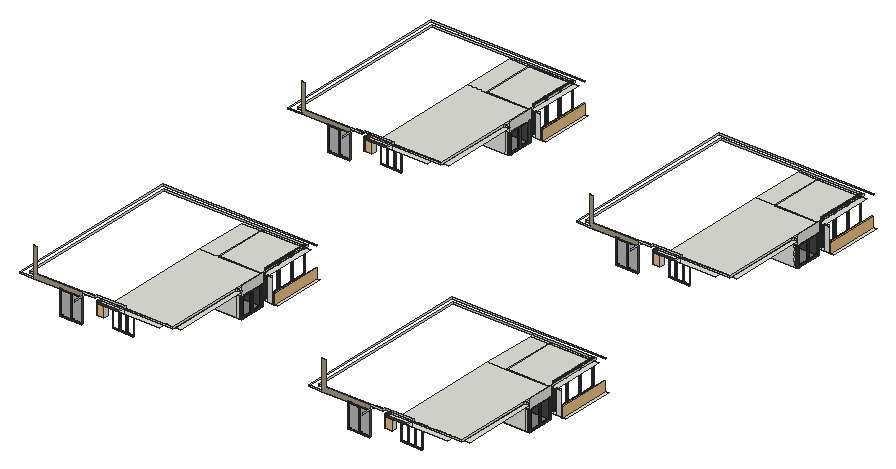
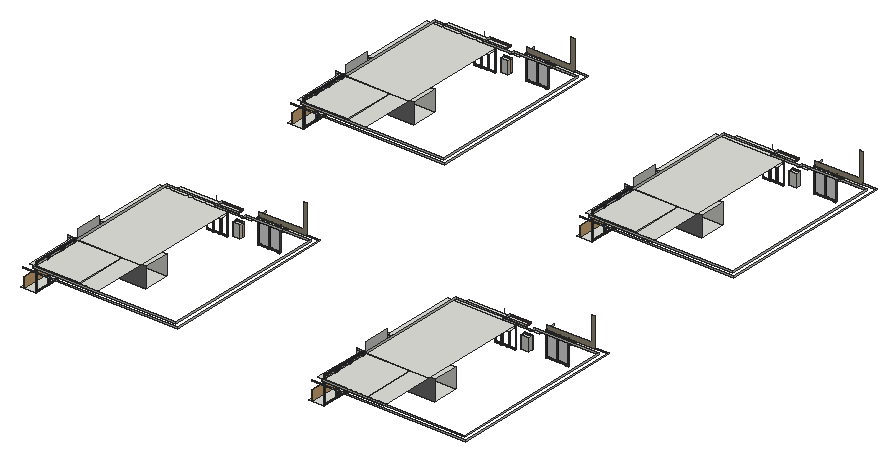
# SketchUp Ruby script. Lengths in inches.
U = 1.inch
M = Sketchup.active_model
def pt(a) = Geom::Point3d.new(a.map { |v| v * U })
def face(e, loops, mat)
  f = e.add_face(loops[0].map { |a| pt(a) })
  loops[1..].each { |l| e.add_face(l.map { |a| pt(a) }).erase! }
  f.material = f.back_material = mat if mat
  f
end
# faces: each face lists its corners as indices into pts; further lists are holes
def faces(e, pts, list, mat = nil) = list.each { |f| face(e, (f[0].is_a?(Array) ? f : [f]).map { |l| l.map { |i| pts[i] } }, mat) }
# xy, xz, yz: faces in a plane at the given z, y or x. An outline is a flat list of corners, or four numbers for a rectangle; further outlines are holes
def ring(l) = l.size == 4 ? [[l[0], l[1]], [l[2], l[1]], [l[2], l[3]], [l[0], l[3]]] : l.each_slice(2).to_a
def flat(e, list, mat, &to3) = list.each { |f| face(e, (f[0].is_a?(Array) ? f : [f]).map { |l| ring(l).map { |u, v| to3.(u, v) } }, mat) }
def xy(e, z, list, mat = nil) = flat(e, list, mat) { |x, y| [x, y, z] }
def xz(e, y, list, mat = nil) = flat(e, list, mat) { |x, z| [x, y, z] }
def yz(e, x, list, mat = nil) = flat(e, list, mat) { |y, z| [x, y, z] }
def lines(e, pts, list) = list.each { |a, b| e.add_line(pt(pts[a]), pt(pts[b])) }
# prism: a flat outline (further loops are holes) pulled along v
def prism(e, loops, v, mat = nil)
  f = face(e, loops, mat); d = Geom::Vector3d.new(v.map { |x| x * U })
  f.pushpull(f.normal.samedirection?(d) ? d.length : -d.length)
end
def box(e, o, s, mat = nil) = prism(e, [[o, [o[0] + s[0], o[1], o[2]], [o[0] + s[0], o[1] + s[1], o[2]], [o[0], o[1] + s[1], o[2]]]], [0, 0, s[2]], mat)
def at(x, y, z, deg = 0) = Geom::Transformation.translation(pt([x, y, z])) * Geom::Transformation.rotation(ORIGIN, Z_AXIS, deg.degrees)
def axes(o, x, y, z) = Geom::Transformation.new([*x, 0, *y, 0, *z, 0, *pt(o).to_a, 1])
def part(name) = M.definitions.add(name)
# library, detail: a bought-in or finely detailed component or shape, given as its bounding box
def library(name, o, s) = part(name).tap { |d| box(d.entities, o, s) }
def detail(e, o, s) = box(e.add_group.entities, o, s)
def put(e, d, t, mat = nil) = e.add_instance(d, t).tap { |i| i.material = mat if mat }
def group(e, t, mat = nil) = e.add_group.tap { |g| g.transformation = t; g.material = mat if mat }.entities
root = M.entities
M.materials.add("Glass_Tinted_Gray").color = [0, 0, 0]
M.materials["Glass_Tinted_Gray"].alpha = 0.125
M.materials.add("Wine2").color = [0, 0, 0]
M.materials["Wine2"].alpha = 0
M.materials.add("[0130_Gainsboro]").color = [39, 45, 50]
M.materials.add("[0135_DarkGray]").color = [81, 81, 81]
M.materials.add("[Color M05]").color = [114, 114, 114]
M.materials.add("[Color M06]").color = [86, 86, 86]
M.materials.add("[Concrete Tile]").color = [165, 155, 133]
M.materials.add("[Granite Brown]").color = [89, 59, 61]
M.materials.add("[Mirror 02]").color = [229, 229, 229]
M.materials.add("[Terrazzo Light Blue]").color = [196, 214, 227]
c1 = part("PENTEK_RP Fineline 50S_Sliding_DoorCase_E1")
box(c1.entities,[0,0,0],[1.51,3.66,99.27],"[0135_DarkGray]")
c2 = part("PENTEK_RP Fineline 50S_SlidingDooe_Case_E2")
box(c2.entities,[0,0,0],[96.25,3.66,1.51],"[0135_DarkGray]")
c3 = part("pentek_RP Fineline 50S_SlidingDoor_Case")
put(c3.entities,c1,at(97.76,0,0))
put(c3.entities,c2,at(1.51,0,0))
put(c3.entities,c1,at(0,0,0))
put(c3.entities,c2,at(1.51,0,97.76))
c4 = part("PENTEK_RP Fineline 50S_SlidingDoor_GlazingBead_2")
box(c4.entities,[0,0,0],[0.56,0.59,94.39],"[0135_DarkGray]")
c5 = part("PENTEK_RP Fineline 50S_SlidingDoor_Glass")
box(c5.entities,[0,0,0],[46.58,0.16,94.39],"Glass_Tinted_Gray")
c6 = part("PENTEK_RP Fineline 50S_SlidingDoor_GlazingBead")
box(c6.entities,[0,0,0],[45.47,0.59,0.56],"[0135_DarkGray]")
c7 = part("PENTEK_RP Fineline 50S_SlidingDoor_Leaf_E1")
xy(c7.entities,0,[[0,0,0.93,1.97],[0.93,1.57,1.49,1.97]],"[0135_DarkGray]")
xy(c7.entities,96.25,[[0,0,0.93,0,0.93,1.57,1.49,1.57,1.49,1.97,0,1.97]],"[0135_DarkGray]")
xz(c7.entities,0,[[0,0,0.93,96.25]],"[0135_DarkGray]")
xz(c7.entities,1.57,[[0.93,0,1.49,95.32],[0.93,95.32,1.49,96.25]],"[0135_DarkGray]")
xz(c7.entities,1.97,[[0,0,1.49,96.25]],"[0135_DarkGray]")
yz(c7.entities,0,[[0,0,1.97,96.25]],"[0135_DarkGray]")
yz(c7.entities,0.93,[[0,0,1.57,0.93],[0,0.93,1.57,95.32],[0,95.32,1.57,96.25]],"[0135_DarkGray]")
yz(c7.entities,1.49,[[1.57,0,1.97,95.32],[1.57,95.32,1.97,96.25]],"[0135_DarkGray]")
c8 = part("PENTEK_RP Fineline 50S_SlidingDoor_Leaf_E2")
xy(c8.entities,0,[[0,0,0,1.57,0.56,1.57,0.56,1.97,46.02,1.97,46.02,1.57,46.58,1.57,46.58,0]],"[0135_DarkGray]")
xy(c8.entities,0.93,[[0,0,46.58,1.57]],"[0135_DarkGray]")
xy(c8.entities,1.49,[[0.56,1.57,46.02,1.97]],"[0135_DarkGray]")
xz(c8.entities,0,[[0,0,46.58,0.93]],"[0135_DarkGray]")
xz(c8.entities,1.57,[[0,0,0.56,0.93],[46.02,0,46.58,0.93],[0.56,0.93,46.02,1.49]],"[0135_DarkGray]")
xz(c8.entities,1.97,[[0.56,0,46.02,1.49]],"[0135_DarkGray]")
yz(c8.entities,0,[[0,0,1.57,0.93]],"[0135_DarkGray]")
yz(c8.entities,0.56,[[1.57,0,1.97,0.93],[1.57,0.93,1.97,1.49]],"[0135_DarkGray]")
yz(c8.entities,46.02,[[1.57,0,1.97,0.93],[1.57,0.93,1.97,1.49]],"[0135_DarkGray]")
yz(c8.entities,46.58,[[0,0,1.57,0.93]],"[0135_DarkGray]")
c9 = part("PENTEK_RP Fineline S_SlidingDoor_Leaf1")
put(c9.entities,c4,at(0.93,0,0.93))
put(c9.entities,c4,at(46.96,0,0.93))
put(c9.entities,c5,at(1.49,1.42,0.93))
put(c9.entities,c6,at(1.49,0,0.93))
put(c9.entities,c5,at(1.49,0.59,0.93),"[Terrazzo Light Blue]")
put(c9.entities,c7,at(0,0,0))
put(c9.entities,c7,axes([48.44,0,0],[-1,0,0],[0,1,0],[0,0,1]))
put(c9.entities,c8,axes([0.93,0,96.25],[1,0,0],[0,1,0],[0,0,-1]))
put(c9.entities,c8,at(0.93,0,0))
put(c9.entities,c6,at(1.49,0,94.77))
c10 = part("PENTEK_RP Fineline 50S_SlidingDoor_Leaf2")
put(c10.entities,c5,at(1.49,1.42,0.93))
put(c10.entities,c6,at(1.49,0,94.77))
put(c10.entities,c4,at(46.96,0,0.93))
put(c10.entities,c5,at(1.49,0.59,0.93),"[Mirror 02]")
put(c10.entities,c4,at(0.93,0,0.93))
put(c10.entities,c7,at(0,0,0))
put(c10.entities,c7,axes([48.44,0,0],[-1,0,0],[0,1,0],[0,0,1]))
put(c10.entities,c6,at(1.49,0,0.93))
put(c10.entities,c8,axes([0.93,0,96.25],[1,0,0],[0,1,0],[0,0,-1]))
put(c10.entities,c8,at(0.93,0,0))
c11 = part("PENTEK - Slimmest Steel Sliding Door / Window\#1")
put(c11.entities,c3,at(0,-1.88,-0.09))
put(c11.entities,c9,at(1.51,-2.27,1.42))
put(c11.entities,c10,at(49.32,-0.3,1.42))
c12 = part("Framed glazing panel")
xy(c12.entities,0,[[0,-0.98,43.07,0],[0,0,43.07,1.4]],"[0130_Gainsboro]")
xy(c12.entities,0.3,[[0.3,-1.43,42.77,-0.98]],"[0130_Gainsboro]")
xy(c12.entities,2.95,[[2.95,-1.43,40.12,-0.63],[2.95,-0.63,40.12,0],[2.95,0,40.12,0.64],[2.95,0.64,40.12,1.4]],"[0130_Gainsboro]")
xy(c12.entities,3.54,[[3.54,-0.63,39.53,0],[3.54,0,39.53,0.64]],"[0130_Gainsboro]")
xy(c12.entities,111.8125,[[3.54,-0.63,39.53,0],[3.54,0,39.53,0.64]],"[0130_Gainsboro]")
xy(c12.entities,112.4,[[2.95,-1.43,40.12,-0.63],[2.95,-0.63,40.12,0],[2.95,0,40.12,0.64],[2.95,0.64,40.12,1.4]],"[0130_Gainsboro]")
xy(c12.entities,115.05,[[0.3,-1.43,42.77,-0.98]],"[0130_Gainsboro]")
xy(c12.entities,115.35,[[0,-0.98,43.07,0],[0,0,43.07,1.4]],"[0130_Gainsboro]")
xz(c12.entities,-1.43,[[[0.3,0.3,42.77,115.05],[2.95,2.95,40.12,112.4]]],"[0130_Gainsboro]")
xz(c12.entities,-0.98,[[[0,0,43.07,115.35],[0.3,0.3,42.77,115.05]]],"[0130_Gainsboro]")
xz(c12.entities,-0.63,[[[2.95,2.95,40.12,112.4],[3.54,3.54,39.53,111.8125]]],"[0130_Gainsboro]")
xz(c12.entities,0,[[3.54,3.54,39.53,111.8125]],"Wine2")
xz(c12.entities,0,[[[0,0,43.07,115.35],[2.95,2.95,40.12,112.4]],[[2.95,2.95,40.12,112.4],[3.54,3.54,39.53,111.8125]]],"[0130_Gainsboro]")
xz(c12.entities,0.64,[[[2.95,2.95,40.12,112.4],[3.54,3.54,39.53,111.8125]]],"[0130_Gainsboro]")
xz(c12.entities,1.4,[[[0,0,43.07,115.35],[2.95,2.95,40.12,112.4]]],"[0130_Gainsboro]")
yz(c12.entities,0,[[-0.98,0,0,115.35],[0,0,1.4,115.35]],"[0130_Gainsboro]")
yz(c12.entities,0.3,[[-1.43,0.3,-0.98,115.05]],"[0130_Gainsboro]")
yz(c12.entities,2.95,[[-1.43,2.95,-0.63,112.4],[-0.63,2.95,0,112.4],[0,2.95,0.64,112.4],[0.64,2.95,1.4,112.4]],"[0130_Gainsboro]")
yz(c12.entities,3.54,[[-0.63,3.54,0,111.8125],[0,3.54,0.64,111.8125]],"[0130_Gainsboro]")
yz(c12.entities,39.53,[[-0.63,3.54,0,111.8125],[0,3.54,0.64,111.8125]],"[0130_Gainsboro]")
yz(c12.entities,40.12,[[-1.43,2.95,-0.63,112.4],[-0.63,2.95,0,112.4],[0,2.95,0.64,112.4],[0.64,2.95,1.4,112.4]],"[0130_Gainsboro]")
yz(c12.entities,42.77,[[-1.43,0.3,-0.98,115.05]],"[0130_Gainsboro]")
yz(c12.entities,43.07,[[-0.98,0,0,115.35],[0,0,1.4,115.35]],"[0130_Gainsboro]")
c13 = part("Glazed panel assembly")
put(c13.entities,c12,axes([90.57,1.43,0],[1.05148,0,0],[0,1,0],[0,0,1]))
put(c13.entities,c12,axes([0,1.43,0],[1.05148,0,0],[0,1,0],[0,0,1]))
put(c13.entities,c12,axes([45.29,1.43,0],[1.05148,0,0],[0,1,0],[0,0,1]))
c14 = library("Glass Railing",[0,0,0],[139.5,4.76,42])
c15 = library("Klein+raam",[128.36,12.7,0],[19.68,5.51,55.12])
xy(root,1409.36,[[625.125,2156.01,913.875,2266.33],[1843.3125,2156.01,2132.0625,2266.33],[625.125,3570.7,913.875,3681.01],[1843.3125,3570.7,2132.0625,3681.01]])
xy(root,1412.8125,[[890.875,2295.875,954.6875,2518.89],[2109.0625,2295.875,2172.875,2518.89],[890.875,3710.5625,954.6875,3933.57],[2109.0625,3710.5625,2172.875,3933.57]])
xy(root,1441.98,[[557.4,1835.1875,588.66,1854.3125],[1775.59,1835.1875,1806.84,1854.3125],[557.4,3249.875,588.66,3269],[1775.59,3249.875,1806.84,3269]])
xy(root,1494.26,[[557.4,1835.1875,588.66,1854.3125],[1775.59,1835.1875,1806.84,1854.3125],[557.4,3249.875,588.66,3269],[1775.59,3249.875,1806.84,3269]])
xy(root,1495.04,[[625.125,2156.01,913.875,2266.33],[1843.3125,2156.01,2132.0625,2266.33],[625.125,3570.7,913.875,3681.01],[1843.3125,3570.7,2132.0625,3681.01]])
xy(root,1502.33,[[625.7,1835.1875,715.63,1873.375],[1843.88,1835.1875,1933.82,1873.375],[625.7,3249.875,715.63,3288.0625],[1843.88,3249.875,1933.82,3288.0625]])
xy(root,1512,[[319.53,1799.9375,319.53,1822.9375,406.18,1822.9375,406.18,1806.5625,431.33,1806.5625,431.33,1822.9375,523.04,1822.9375,523.04,1799.9375],[589.7,1799.9375,679.51,1822.9375],[679.51,1799.9375,851.78,1822.9375],[1537.72,1799.9375,1537.72,1822.9375,1624.37,1822.9375,1624.37,1806.5625,1649.52,1806.5625,1649.52,1822.9375,1741.23,1822.9375,1741.23,1799.9375],[1807.88,1799.9375,1897.7,1822.9375],
  [1897.7,1799.9375,2069.97,1822.9375],[523.04,1822.9375,557.4,1836.125],[679.51,1822.9375,851.78,1835.1875],[851.78,1822.9375,890.875,1835.1875],[1741.23,1822.9375,1775.59,1836.125],
  [1897.7,1822.9375,2069.97,1835.1875],[2069.97,1822.9375,2109.0625,1835.1875],[557.4,1835.1875,625.125,1836.125],[625.125,1835.1875,890.875,2295.875],[894.3125,1835.1875,913.875,2156.01],
  [1775.59,1835.1875,1843.3125,1836.125],[1843.3125,1835.1875,2109.0625,2295.875],[2112.5,1835.1875,2132.0625,2156.01],[625.125,2295.875,704.25,2518.89],[704.25,2295.875,890.875,2518.89],
  [890.875,2295.875,913.875,2518.89],[1843.3125,2295.875,1922.4375,2518.89],[1922.4375,2295.875,2109.0625,2518.89],[2109.0625,2295.875,2132.0625,2518.89],[625.125,2518.89,890.875,2531.375],
  [1843.3125,2518.89,2109.0625,2531.375],[319.53,3214.625,319.53,3237.625,406.18,3237.625,406.18,3221.25,431.33,3221.25,431.33,3237.625,523.04,3237.625,523.04,3214.625],[589.7,3214.625,679.51,3237.625],[679.51,3214.625,851.78,3237.625],[1537.72,3214.625,1537.72,3237.625,1624.37,3237.625,1624.37,3221.25,1649.52,3221.25,1649.52,3237.625,1741.23,3237.625,1741.23,3214.625],
  [1807.88,3214.625,1897.7,3237.625],[1897.7,3214.625,2069.97,3237.625],[523.04,3237.625,557.4,3250.8125],[679.51,3237.625,851.78,3249.875],[851.78,3237.625,890.875,3249.875],
  [1741.23,3237.625,1775.59,3250.8125],[1897.7,3237.625,2069.97,3249.875],[2069.97,3237.625,2109.0625,3249.875],[557.4,3249.875,625.125,3250.8125],[625.125,3249.875,890.875,3710.5625],
  [894.3125,3249.875,913.875,3570.7],[1775.59,3249.875,1843.3125,3250.8125],[1843.3125,3249.875,2109.0625,3710.5625],[2112.5,3249.875,2132.0625,3570.7],[625.125,3710.5625,704.25,3933.57],
  [704.25,3710.5625,890.875,3933.57],[890.875,3710.5625,913.875,3933.57],[1843.3125,3710.5625,1922.4375,3933.57],[1922.4375,3710.5625,2109.0625,3933.57],[2109.0625,3710.5625,2132.0625,3933.57],
  [625.125,3933.57,890.875,3946.0625],[1843.3125,3933.57,2109.0625,3946.0625]])
xy(root,1512,[[557.4,1822.9375,557.88,1835.1875],[1775.59,1822.9375,1776.07,1835.1875],[557.4,3237.625,557.88,3249.875],[1775.59,3237.625,1776.07,3249.875]],"[Granite Brown]")
xy(root,1513.25,[[704.25,2295.875,890.875,2518.89],[1922.4375,2295.875,2109.0625,2518.89],[704.25,3710.5625,890.875,3933.57],[1922.4375,3710.5625,2109.0625,3933.57]])
xz(root,1799.9375,[[262.875,1512,319.53,1518],[1481.0625,1512,1537.72,1518]])
xz(root,1799.9375,[[319.53,1512,523.04,1512,523.04,1533.4375,333.68,1533.4375,333.68,1638,319.53,1638],[1537.72,1512,1741.23,1512,1741.23,1533.4375,1551.87,1533.4375,1551.87,1638,1537.72,1638]],"[Concrete Tile]")
xz(root,1799.9375,[[589.7,1512,679.51,1518],[1807.88,1512,1897.7,1518]],"[Granite Brown]")
xz(root,1822.9375,[[285.875,1512,285.875,1518,557.4,1518,557.4,1512,406.18,1512,395.37,1512.05,395.37,1512],[395.37,1512,395.37,1512.05,406.18,1512],[589.7,1512,679.51,1518],[679.51,1512,890.875,1518],[1504.0625,1512,1504.0625,1518,1775.59,1518,1775.59,1512,1624.37,1512,1613.56,1512.05,1613.56,1512],
  [1613.56,1512,1613.56,1512.05,1624.37,1512],[1807.88,1512,1897.7,1518],[1897.7,1512,2109.0625,1518]])
xz(root,1822.9375,[[557.4,1512,557.88,1518],[1775.59,1512,1776.07,1518]],"[Granite Brown]")
xz(root,1835.1875,[[556.34,1441.98,557.4,1494.26],[1774.53,1441.98,1775.59,1494.26],[557.4,1512,679.51,1518],[1775.59,1512,1897.7,1518]])
xz(root,1835.1875,[[557.4,1441.98,557.88,1494.26],[1775.59,1441.98,1776.07,1494.26]],"[Granite Brown]")
xz(root,1854.3125,[[557.4,1441.98,588.66,1494.26],[1775.59,1441.98,1806.84,1494.26]])
xz(root,2156.01,[[625.125,1409.36,894.3125,1495.04],[894.3125,1409.36,913.875,1495.04],[1843.3125,1409.36,2112.5,1495.04],[2112.5,1409.36,2132.0625,1495.04],[894.3125,1495.04,913.875,1512],
  [2112.5,1495.04,2132.0625,1512],[894.3125,1512,913.875,1518],[2112.5,1512,2132.0625,1518]])
xz(root,2266.33,[[625.125,1409.36,913.875,1495.04],[1843.3125,1409.36,2132.0625,1495.04]],"[Color M05]")
xz(root,2295.875,[[913.875,1412.8125,930.75,1512],[2132.0625,1412.8125,2148.9375,1512],[704.25,1512,890.875,1513.25],[913.875,1512,930.75,1518],[1922.4375,1512,2109.0625,1513.25],
  [2132.0625,1512,2148.9375,1518]])
xz(root,2518.89,[[704.25,1512,890.875,1513.25],[1922.4375,1512,2109.0625,1513.25]])
xz(root,2531.375,[[285.875,1512,890.875,1518],[1504.0625,1512,2109.0625,1518]])
xz(root,2554.375,[[262.875,1512,913.875,1518],[1481.0625,1512,2132.0625,1518]])
xz(root,3214.625,[[262.875,1512,319.53,1518],[1481.0625,1512,1537.72,1518]])
xz(root,3214.625,[[319.53,1512,523.04,1512,523.04,1533.4375,333.68,1533.4375,333.68,1638,319.53,1638],[1537.72,1512,1741.23,1512,1741.23,1533.4375,1551.87,1533.4375,1551.87,1638,1537.72,1638]],"[Concrete Tile]")
xz(root,3214.625,[[589.7,1512,679.51,1518],[1807.88,1512,1897.7,1518]],"[Granite Brown]")
xz(root,3237.625,[[285.875,1512,285.875,1518,557.4,1518,557.4,1512,406.18,1512,395.37,1512.05,395.37,1512],[395.37,1512,395.37,1512.05,406.18,1512],[589.7,1512,679.51,1518],[679.51,1512,890.875,1518],[1504.0625,1512,1504.0625,1518,1775.59,1518,1775.59,1512,1624.37,1512,1613.56,1512.05,1613.56,1512],
  [1613.56,1512,1613.56,1512.05,1624.37,1512],[1807.88,1512,1897.7,1518],[1897.7,1512,2109.0625,1518]])
xz(root,3237.625,[[557.4,1512,557.88,1518],[1775.59,1512,1776.07,1518]],"[Granite Brown]")
xz(root,3249.875,[[556.34,1441.98,557.4,1494.26],[1774.53,1441.98,1775.59,1494.26],[557.4,1512,679.51,1518],[1775.59,1512,1897.7,1518]])
xz(root,3249.875,[[557.4,1441.98,557.88,1494.26],[1775.59,1441.98,1776.07,1494.26]],"[Granite Brown]")
xz(root,3269,[[557.4,1441.98,588.66,1494.26],[1775.59,1441.98,1806.84,1494.26]])
xz(root,3570.7,[[625.125,1409.36,894.3125,1495.04],[894.3125,1409.36,913.875,1495.04],[1843.3125,1409.36,2112.5,1495.04],[2112.5,1409.36,2132.0625,1495.04],[894.3125,1495.04,913.875,1512],
  [2112.5,1495.04,2132.0625,1512],[894.3125,1512,913.875,1518],[2112.5,1512,2132.0625,1518]])
xz(root,3681.01,[[625.125,1409.36,913.875,1495.04],[1843.3125,1409.36,2132.0625,1495.04]],"[Color M05]")
xz(root,3710.5625,[[913.875,1412.8125,930.75,1512],[2132.0625,1412.8125,2148.9375,1512],[704.25,1512,890.875,1513.25],[913.875,1512,930.75,1518],[1922.4375,1512,2109.0625,1513.25],
  [2132.0625,1512,2148.9375,1518]])
xz(root,3933.57,[[704.25,1512,890.875,1513.25],[1922.4375,1512,2109.0625,1513.25]])
xz(root,3946.0625,[[285.875,1512,890.875,1518],[1504.0625,1512,2109.0625,1518]])
xz(root,3969.0625,[[262.875,1512,913.875,1518],[1481.0625,1512,2132.0625,1518]])
yz(root,262.875,[[1799.9375,1512,2554.375,1518],[3214.625,1512,3969.0625,1518]])
yz(root,285.875,[[1822.9375,1512,2531.375,1518],[3237.625,1512,3946.0625,1518]])
yz(root,523.04,[[1763.25,1512,1799.9375,1518],[3177.9375,1512,3214.625,1518]])
yz(root,557.4,[[1835.1875,1441.98,1854.3125,1494.26],[3249.875,1441.98,3269,1494.26],[1822.9375,1512,1835.1875,1518],[3237.625,1512,3249.875,1518]])
yz(root,588.66,[[1835.1875,1441.98,1854.3125,1494.26],[3249.875,1441.98,3269,1494.26]])
yz(root,589.7,[[1799.9375,1512,1822.9375,1518],[3214.625,1512,3237.625,1518]],"[Granite Brown]")
yz(root,679.51,[[1799.9375,1512,1822.9375,1518],[1822.9375,1512,1835.1875,1518],[3214.625,1512,3237.625,1518],[3237.625,1512,3249.875,1518]])
yz(root,704.25,[[2295.875,1512,2518.89,1513.25],[3710.5625,1512,3933.57,1513.25]])
yz(root,890.875,[[1822.9375,1512,1822.9375,1518,2531.375,1518,2531.375,1512,2518.89,1512,2518.89,1513.25,2295.875,1513.25,2295.875,1512],[2295.875,1512,2518.89,1513.25],[3237.625,1512,3237.625,1518,3946.0625,1518,3946.0625,1512,3933.57,1512,3933.57,1513.25,3710.5625,1513.25,3710.5625,1512],[3710.5625,1512,3933.57,1513.25]])
yz(root,894.3125,[[2148.83,1512,2156.01,1518],[3563.51,1512,3570.7,1518]])
yz(root,913.875,[[2156.01,1495.04,2266.33,1535.36],[3570.7,1495.04,3681.01,1535.36],[2148.83,1512,2156.01,1518],[3563.51,1512,3570.7,1518]])
yz(root,1481.0625,[[1799.9375,1512,2554.375,1518],[3214.625,1512,3969.0625,1518]])
yz(root,1504.0625,[[1822.9375,1512,2531.375,1518],[3237.625,1512,3946.0625,1518]])
yz(root,1741.23,[[1763.25,1512,1799.9375,1518],[3177.9375,1512,3214.625,1518]])
yz(root,1775.59,[[1835.1875,1441.98,1854.3125,1494.26],[3249.875,1441.98,3269,1494.26],[1822.9375,1512,1835.1875,1518],[3237.625,1512,3249.875,1518]])
yz(root,1806.84,[[1835.1875,1441.98,1854.3125,1494.26],[3249.875,1441.98,3269,1494.26]])
yz(root,1807.88,[[1799.9375,1512,1822.9375,1518],[3214.625,1512,3237.625,1518]],"[Granite Brown]")
yz(root,1897.7,[[1799.9375,1512,1822.9375,1518],[1822.9375,1512,1835.1875,1518],[3214.625,1512,3237.625,1518],[3237.625,1512,3249.875,1518]])
yz(root,1922.4375,[[2295.875,1512,2518.89,1513.25],[3710.5625,1512,3933.57,1513.25]])
yz(root,2109.0625,[[1822.9375,1512,1822.9375,1518,2531.375,1518,2531.375,1512,2518.89,1512,2518.89,1513.25,2295.875,1513.25,2295.875,1512],[2295.875,1512,2518.89,1513.25],[3237.625,1512,3237.625,1518,3946.0625,1518,3946.0625,1512,3933.57,1512,3933.57,1513.25,3710.5625,1513.25,3710.5625,1512],[3710.5625,1512,3933.57,1513.25]])
yz(root,2112.5,[[2148.83,1512,2156.01,1518],[3563.51,1512,3570.7,1518]])
yz(root,2132.0625,[[2156.01,1495.04,2266.33,1535.36],[3570.7,1495.04,3681.01,1535.36],[2148.83,1512,2156.01,1518],[3563.51,1512,3570.7,1518]])
p = [[406.18,1806.5625,1512],[406.18,1822.9375,1512],[395.37,1822.9375,1512.05],[395.37,1806.5625,1512.05],[1624.37,1806.5625,1512],[1624.37,1822.9375,1512],
  [1613.56,1822.9375,1512.05],[1613.56,1806.5625,1512.05],[406.18,3221.25,1512],[406.18,3237.625,1512],[395.37,3237.625,1512.05],[395.37,3221.25,1512.05],
  [1624.37,3221.25,1512],[1624.37,3237.625,1512],[1613.56,3237.625,1512.05],[1613.56,3221.25,1512.05],[1919.95,1800.76,1530.58],[1920.14,1799.9375,1512],
  [701.76,1800.76,1530.58],[701.96,1799.9375,1512],[1919.95,3215.45,1530.58],[1920.14,3214.625,1512],[701.76,3215.45,1530.58],[701.96,3214.625,1512]]
faces(root,p,[[0,1,2,3],[4,5,6,7],[8,9,10,11],[12,13,14,15]])
lines(root,p,[[16,17],[18,19],[20,21],[22,23]])
put(root,c11,axes([1647.8,1801.54,1408.78],[0.94111,0,0],[0,0.88,0],[0,0,1.054]))
put(root,c11,axes([429.61,1801.54,1408.78],[0.94111,0,0],[0,0.88,0],[0,0,1.054]))
put(root,c11,axes([1647.8,3216.23,1408.78],[0.94111,0,0],[0,0.88,0],[0,0,1.054]))
put(root,c11,axes([429.61,3216.23,1408.78],[0.94111,0,0],[0,0.88,0],[0,0,1.054]))
put(root,c11,axes([2127.34,2156.65,1409.4375],[0,1.12181,0],[-2.51374,0,0],[0,0,0.87918]))
put(root,c11,axes([909.16,2156.65,1409.4375],[0,1.12181,0],[-2.51374,0,0],[0,0,0.87918]))
put(root,c11,axes([2127.34,3571.34,1409.4375],[0,1.12181,0],[-2.51374,0,0],[0,0,0.87918]))
put(root,c11,axes([909.16,3571.34,1409.4375],[0,1.12181,0],[-2.51374,0,0],[0,0,0.87918]))
put(root,c13,axes([2109.0625,2310.05,1412.51],[0,1.54079,0],[-1,0,0],[0,0,1]))
put(root,c13,axes([890.875,2310.05,1412.51],[0,1.54079,0],[-1,0,0],[0,0,1]))
put(root,c13,axes([2109.0625,3724.73,1412.51],[0,1.54079,0],[-1,0,0],[0,0,1]))
put(root,c13,axes([890.875,3724.73,1412.51],[0,1.54079,0],[-1,0,0],[0,0,1]))
put(root,c14,axes([2159.4375,2295.6875,1412.8125],[0,1.6,0],[-1,0,0],[0,0,1]))
put(root,c14,axes([941.25,2295.6875,1412.8125],[0,1.6,0],[-1,0,0],[0,0,1]))
put(root,c14,axes([2159.4375,3710.375,1412.8125],[0,1.6,0],[-1,0,0],[0,0,1]))
put(root,c14,axes([941.25,3710.375,1412.8125],[0,1.6,0],[-1,0,0],[0,0,1]))
put(root,c13,axes([1843.49,1833.46,1415.83],[0.6649,0,0],[0,0.61,0],[0,0,0.74986]),"[Color M06]")
put(root,c13,axes([625.3,1833.46,1415.83],[0.6649,0,0],[0,0.61,0],[0,0,0.74986]),"[Color M06]")
put(root,c13,axes([1843.49,3248.15,1415.83],[0.6649,0,0],[0,0.61,0],[0,0,0.74986]),"[Color M06]")
put(root,c13,axes([625.3,3248.15,1415.83],[0.6649,0,0],[0,0.61,0],[0,0,0.74986]),"[Color M06]")
put(root,c15,axes([1571.78,1826.29,1442.29],[1.58777,0,0],[0,0.68,0],[0,0,0.99202]))
put(root,c15,axes([353.6,1826.29,1442.29],[1.58777,0,0],[0,0.68,0],[0,0,0.99202]))
put(root,c15,axes([1571.78,3240.97,1442.29],[1.58777,0,0],[0,0.68,0],[0,0,0.99202]))
put(root,c15,axes([353.6,3240.97,1442.29],[1.58777,0,0],[0,0.68,0],[0,0,0.99202]))
